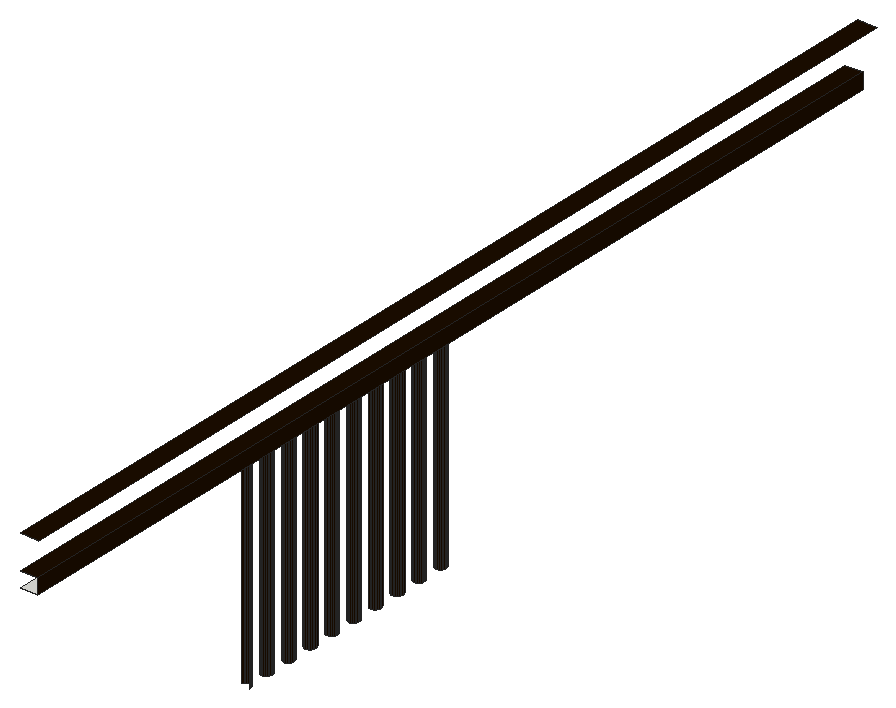
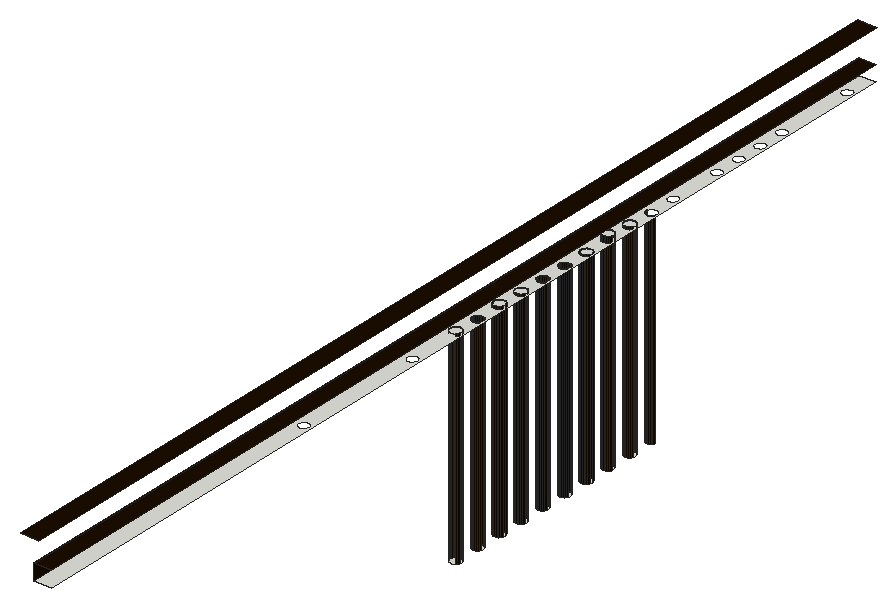
# SketchUp Ruby script. Lengths in inches.
U = 1.inch
M = Sketchup.active_model
def pt(a) = Geom::Point3d.new(a.map { |v| v * U })
def face(e, loops, mat)
  f = e.add_face(loops[0].map { |a| pt(a) })
  loops[1..].each { |l| e.add_face(l.map { |a| pt(a) }).erase! }
  f.material = f.back_material = mat if mat
  f
end
# faces: each face lists its corners as indices into pts; further lists are holes
def faces(e, pts, list, mat = nil) = list.each { |f| face(e, (f[0].is_a?(Array) ? f : [f]).map { |l| l.map { |i| pts[i] } }, mat) }
# xy, xz, yz: faces in a plane at the given z, y or x. An outline is a flat list of corners, or four numbers for a rectangle; further outlines are holes
def ring(l) = l.size == 4 ? [[l[0], l[1]], [l[2], l[1]], [l[2], l[3]], [l[0], l[3]]] : l.each_slice(2).to_a
def flat(e, list, mat, &to3) = list.each { |f| face(e, (f[0].is_a?(Array) ? f : [f]).map { |l| ring(l).map { |u, v| to3.(u, v) } }, mat) }
def xy(e, z, list, mat = nil) = flat(e, list, mat) { |x, y| [x, y, z] }
def xz(e, y, list, mat = nil) = flat(e, list, mat) { |x, z| [x, y, z] }
def yz(e, x, list, mat = nil) = flat(e, list, mat) { |y, z| [x, y, z] }
def lines(e, pts, list) = list.each { |a, b| e.add_line(pt(pts[a]), pt(pts[b])) }
# prism: a flat outline (further loops are holes) pulled along v
def prism(e, loops, v, mat = nil)
  f = face(e, loops, mat); d = Geom::Vector3d.new(v.map { |x| x * U })
  f.pushpull(f.normal.samedirection?(d) ? d.length : -d.length)
end
def box(e, o, s, mat = nil) = prism(e, [[o, [o[0] + s[0], o[1], o[2]], [o[0] + s[0], o[1] + s[1], o[2]], [o[0], o[1] + s[1], o[2]]]], [0, 0, s[2]], mat)
def at(x, y, z, deg = 0) = Geom::Transformation.translation(pt([x, y, z])) * Geom::Transformation.rotation(ORIGIN, Z_AXIS, deg.degrees)
def axes(o, x, y, z) = Geom::Transformation.new([*x, 0, *y, 0, *z, 0, *pt(o).to_a, 1])
def part(name) = M.definitions.add(name)
# library, detail: a bought-in or finely detailed component or shape, given as its bounding box
def library(name, o, s) = part(name).tap { |d| box(d.entities, o, s) }
def detail(e, o, s) = box(e.add_group.entities, o, s)
def put(e, d, t, mat = nil) = e.add_instance(d, t).tap { |i| i.material = mat if mat }
def group(e, t, mat = nil) = e.add_group.tap { |g| g.transformation = t; g.material = mat if mat }.entities
root = M.entities
M.materials.add("[Metal Seamed]1").color = [28, 14, 0]
xy(root,618.25,[[363.55,142.79,363.21,142.87,362.92,143.04,362.67,143.28,362.5,143.58,362.41,143.91,362.41,144.25,362.5,144.58,362.67,144.88,362.91,145.125,363.2,145.3,363.54,145.39,363.88,145.39,364.21,145.3,364.51,145.13,364.75,144.89,364.92,144.59,365.01,144.26,365.01,143.92,364.93,143.59,364.76,143.29,364.51,143.05,364.22,142.875,363.89,142.79],[363.55,149.22,363.21,149.31,362.92,149.48,362.67,149.72,362.5,150.02,362.41,150.35,362.41,150.69,362.5,151.02,362.67,151.32,362.91,151.5625,363.2,151.74,363.54,151.83,363.88,151.83,364.21,151.74,364.51,151.57,364.75,151.33,364.92,151.03,365.01,150.7,365.01,150.36,364.93,150.03,364.76,149.73,364.51,149.49,364.22,149.3125,363.89,149.22],[363.55,155.66,363.21,155.75,362.92,155.92,362.67,156.16,362.5,156.46,362.41,156.79,362.41,157.13,362.5,157.46,362.67,157.76,362.91,158,363.2,158.17,363.54,158.26,363.88,158.26,364.21,158.18,364.51,158.01,364.75,157.76,364.92,157.47,365.01,157.14,365.01,156.8,364.93,156.46,364.76,156.17,364.51,155.92,364.22,155.75,363.89,155.66],[363.55,162.1,363.21,162.19,362.92,162.36,362.67,162.6,362.5,162.89,362.41,163.22,362.41,163.57,362.5,163.9,362.67,164.19,362.91,164.4375,363.2,164.61,363.54,164.7,363.88,164.7,364.21,164.61,364.51,164.44,364.75,164.2,364.92,163.91,365.01,163.58,365.01,163.23,364.93,162.9,364.76,162.6,364.51,162.36,364.22,162.1875,363.89,162.1],[363.55,168.54,363.21,168.62,362.92,168.79,362.67,169.03,362.5,169.33,362.41,169.66,362.41,170,362.5,170.33,362.67,170.63,362.91,170.875,363.2,171.05,363.54,171.14,363.88,171.14,364.21,171.05,364.51,170.88,364.75,170.64,364.92,170.34,365.01,170.01,365.01,169.67,364.93,169.34,364.76,169.04,364.51,168.8,364.22,168.625,363.89,168.54],
  [363.55,174.97,363.21,175.06,362.92,175.23,362.67,175.47,362.5,175.77,362.41,176.1,362.41,176.44,362.5,176.77,362.67,177.07,362.91,177.3125,363.2,177.49,363.54,177.58,363.88,177.58,364.21,177.49,364.51,177.32,364.75,177.08,364.92,176.78,365.01,176.45,365.01,176.11,364.93,175.78,364.76,175.48,364.51,175.24,364.22,175.0625,363.89,174.97],[363.55,181.41,363.21,181.5,362.92,181.67,362.67,181.91,362.5,182.21,362.41,182.54,362.41,182.88,362.5,183.21,362.67,183.51,362.91,183.75,363.2,183.92,363.54,184.01,363.88,184.01,364.21,183.93,364.51,183.76,364.75,183.51,364.92,183.22,365.01,182.89,365.01,182.55,364.93,182.21,364.76,181.92,364.51,181.67,364.22,181.5,363.89,181.41],[363.55,187.85,363.21,187.94,362.92,188.11,362.67,188.35,362.5,188.64,362.41,188.97,362.41,189.32,362.5,189.65,362.67,189.94,362.91,190.1875,363.2,190.36,363.54,190.45,363.88,190.45,364.21,190.36,364.51,190.19,364.75,189.95,364.92,189.66,365.01,189.33,365.01,188.98,364.93,188.65,364.76,188.35,364.51,188.11,364.22,187.9375,363.89,187.85],[363.55,194.29,363.21,194.37,362.92,194.54,362.67,194.78,362.5,195.08,362.41,195.41,362.41,195.75,362.5,196.08,362.67,196.38,362.91,196.625,363.2,196.8,363.54,196.89,363.88,196.89,364.21,196.8,364.51,196.63,364.75,196.39,364.92,196.09,365.01,195.76,365.01,195.42,364.93,195.09,364.76,194.79,364.51,194.55,364.22,194.375,363.89,194.29]])
xy(root,666.66,[[[361.98,73.28,366.15,317.52],[363.55,78.41,363.89,78.41,364.22,78.5,364.51,78.67,364.76,78.92,364.93,79.21,365.01,79.55,365.01,79.89,364.92,80.22,364.75,80.51,364.51,80.76,364.21,80.93,363.88,81.01,363.54,81.01,363.2,80.92,362.91,80.75,362.67,80.51,362.5,80.21,362.41,79.88,362.41,79.54,362.5,79.21,362.67,78.91,362.92,78.67,363.21,78.5],[363.55,97.72,363.89,97.72,364.22,97.8125,364.51,97.99,364.76,98.23,364.93,98.53,365.01,98.86,365.01,99.2,364.92,99.53,364.75,99.83,364.51,100.07,364.21,100.24,363.88,100.33,363.54,100.33,363.2,100.24,362.91,100.0625,362.67,99.82,362.5,99.52,362.41,99.19,362.41,98.85,362.5,98.52,362.67,98.22,362.92,97.98,363.21,97.81],[363.55,104.16,363.89,104.16,364.22,104.25,364.51,104.42,364.76,104.67,364.93,104.96,365.01,105.3,365.01,105.64,364.92,105.97,364.75,106.26,364.51,106.51,364.21,106.68,363.88,106.76,363.54,106.76,363.2,106.67,362.91,106.5,362.67,106.26,362.5,105.96,362.41,105.63,362.41,105.29,362.5,104.96,362.67,104.66,362.92,104.42,363.21,104.25],[363.55,110.6,363.89,110.6,364.22,110.6875,364.51,110.86,364.76,111.1,364.93,111.4,365.01,111.73,365.01,112.08,364.92,112.41,364.75,112.7,364.51,112.94,364.21,113.11,363.88,113.2,363.54,113.2,363.2,113.11,362.91,112.9375,362.67,112.69,362.5,112.4,362.41,112.07,362.41,111.72,362.5,111.39,362.67,111.1,362.92,110.86,363.21,110.69],[363.55,117.04,363.89,117.04,364.22,117.125,364.51,117.3,364.76,117.54,364.93,117.84,365.01,118.17,365.01,118.51,364.92,118.84,364.75,119.14,364.51,119.38,364.21,119.55,363.88,119.64,363.54,119.64,363.2,119.55,362.91,119.375,362.67,119.13,362.5,118.83,362.41,118.5,362.41,118.16,362.5,117.83,362.67,117.53,362.92,117.29,363.21,117.12],[363.55,129.91,363.89,129.91,364.22,130,364.51,130.17,364.76,130.42,364.93,130.71,365.01,131.05,365.01,131.39,364.92,131.72,364.75,132.01,364.51,132.26,364.21,132.43,363.88,132.51,363.54,132.51,363.2,132.42,362.91,132.25,362.67,132.01,362.5,131.71,362.41,131.38,362.41,131.04,362.5,130.71,362.67,130.41,362.92,130.17,363.21,130],[363.55,136.35,363.89,136.35,364.22,136.4375,364.51,136.61,364.76,136.85,364.93,137.15,365.01,137.48,365.01,137.83,364.92,138.16,364.75,138.45,364.51,138.69,364.21,138.86,363.88,138.95,363.54,138.95,363.2,138.86,362.91,138.6875,362.67,138.44,362.5,138.15,362.41,137.82,362.41,137.47,362.5,137.14,362.67,136.85,362.92,136.61,363.21,136.44],[363.55,162.1,363.89,162.1,364.22,162.1875,364.51,162.36,364.76,162.6,364.93,162.9,365.01,163.23,365.01,163.58,364.92,163.91,364.75,164.2,364.51,164.44,364.21,164.61,363.88,164.7,363.54,164.7,363.2,164.61,362.91,164.4375,362.67,164.19,362.5,163.9,362.41,163.57,362.41,163.22,362.5,162.89,362.67,162.6,362.92,162.36,363.21,162.19],[363.55,168.54,363.89,168.54,364.22,168.625,364.51,168.8,364.76,169.04,364.93,169.34,365.01,169.67,365.01,170.01,364.92,170.34,364.75,170.64,364.51,170.88,364.21,171.05,363.88,171.14,363.54,171.14,363.2,171.05,362.91,170.875,362.67,170.63,362.5,170.33,362.41,170,362.41,169.66,362.5,169.33,362.67,169.03,362.92,168.79,363.21,168.62],[363.55,187.85,363.89,187.85,364.22,187.9375,364.51,188.11,364.76,188.35,364.93,188.65,365.01,188.98,365.01,189.33,364.92,189.66,364.75,189.95,364.51,190.19,364.21,190.36,363.88,190.45,363.54,190.45,363.2,190.36,362.91,190.1875,362.67,189.94,362.5,189.65,362.41,189.32,362.41,188.97,362.5,188.64,362.67,188.35,362.92,188.11,363.21,187.94],[363.55,207.16,363.89,207.16,364.22,207.25,364.51,207.42,364.76,207.67,364.93,207.96,365.01,208.3,365.01,208.64,364.92,208.97,364.75,209.26,364.51,209.51,364.21,209.68,363.88,209.76,363.54,209.76,363.2,209.67,362.91,209.5,362.67,209.26,362.5,208.96,362.41,208.63,362.41,208.29,362.5,207.96,362.67,207.66,362.92,207.42,363.21,207.25],[363.55,239.35,363.89,239.35,364.22,239.4375,364.51,239.61,364.76,239.85,364.93,240.15,365.01,240.48,365.01,240.83,364.92,241.16,364.75,241.45,364.51,241.69,364.21,241.86,363.88,241.95,363.54,241.95,363.2,241.86,362.91,241.6875,362.67,241.44,362.5,241.15,362.41,240.82,362.41,240.47,362.5,240.14,362.67,239.85,362.92,239.61,363.21,239.44]]])
xy(root,666.8125,[[363.55,155.66,363.89,155.66,364.22,155.75,364.51,155.92,364.76,156.17,364.93,156.46,365.01,156.8,365.01,157.14,364.92,157.47,364.75,157.76,364.51,158.01,364.21,158.18,363.88,158.26,363.54,158.26,363.2,158.17,362.91,158,362.67,157.76,362.5,157.46,362.41,157.13,362.41,156.79,362.5,156.46,362.67,156.16,362.92,155.92,363.21,155.75]])
xy(root,667,[[363.55,174.97,363.89,174.97,364.22,175.0625,364.51,175.24,364.76,175.48,364.93,175.78,365.01,176.11,365.01,176.45,364.92,176.78,364.75,177.08,364.51,177.32,364.21,177.49,363.88,177.58,363.54,177.58,363.2,177.49,362.91,177.3125,362.67,177.07,362.5,176.77,362.41,176.44,362.41,176.1,362.5,175.77,362.67,175.47,362.92,175.23,363.21,175.06]])
xy(root,667.125,[[363.55,142.79,363.89,142.79,364.22,142.875,364.51,143.05,364.76,143.29,364.93,143.59,365.01,143.92,365.01,144.26,364.92,144.59,364.75,144.89,364.51,145.13,364.21,145.3,363.88,145.39,363.54,145.39,363.2,145.3,362.91,145.125,362.67,144.88,362.5,144.58,362.41,144.25,362.41,143.91,362.5,143.58,362.67,143.28,362.92,143.04,363.21,142.87],[363.55,194.29,363.89,194.29,364.22,194.375,364.51,194.55,364.76,194.79,364.93,195.09,365.01,195.42,365.01,195.76,364.92,196.09,364.75,196.39,364.51,196.63,364.21,196.8,363.88,196.89,363.54,196.89,363.2,196.8,362.91,196.625,362.67,196.38,362.5,196.08,362.41,195.75,362.41,195.41,362.5,195.08,362.67,194.78,362.92,194.54,363.21,194.37]])
xy(root,667.25,[[363.55,181.41,363.89,181.41,364.22,181.5,364.51,181.67,364.76,181.92,364.93,182.21,365.01,182.55,365.01,182.89,364.92,183.22,364.75,183.51,364.51,183.76,364.21,183.93,363.88,184.01,363.54,184.01,363.2,183.92,362.91,183.75,362.67,183.51,362.5,183.21,362.41,182.88,362.41,182.54,362.5,182.21,362.67,181.91,362.92,181.67,363.21,181.5]])
xy(root,667.9375,[[363.55,149.22,363.89,149.22,364.22,149.3125,364.51,149.49,364.76,149.73,364.93,150.03,365.01,150.36,365.01,150.7,364.92,151.03,364.75,151.33,364.51,151.57,364.21,151.74,363.88,151.83,363.54,151.83,363.2,151.74,362.91,151.5625,362.67,151.32,362.5,151.02,362.41,150.69,362.41,150.35,362.5,150.02,362.67,149.72,362.92,149.48,363.21,149.31]])
xy(root,670.37,[[361.98,73.28,366.15,317.52]],"[Metal Seamed]1")
xy(root,678.3125,[[361.97,73.28,366.34,321.28]],"[Metal Seamed]1")
xz(root,138.95,[[363.54,618.25,363.88,666.66]],"[Metal Seamed]1")
xz(root,142.79,[[363.55,618.25,363.89,667.125]],"[Metal Seamed]1")
xz(root,145.39,[[363.54,618.25,363.88,667.125]],"[Metal Seamed]1")
xz(root,149.22,[[363.55,618.25,363.89,667.9375]],"[Metal Seamed]1")
xz(root,151.83,[[363.54,618.25,363.88,667.9375]],"[Metal Seamed]1")
xz(root,155.66,[[363.55,618.25,363.89,666.8125]],"[Metal Seamed]1")
xz(root,158.26,[[363.54,618.25,363.88,666.8125]],"[Metal Seamed]1")
xz(root,162.1,[[363.55,618.25,363.89,666.66]],"[Metal Seamed]1")
xz(root,164.7,[[363.54,618.25,363.88,666.66]],"[Metal Seamed]1")
xz(root,168.54,[[363.55,618.25,363.89,666.66]],"[Metal Seamed]1")
xz(root,171.14,[[363.54,618.25,363.88,666.66]],"[Metal Seamed]1")
xz(root,174.97,[[363.55,618.25,363.89,667]],"[Metal Seamed]1")
xz(root,177.58,[[363.54,618.25,363.88,667]],"[Metal Seamed]1")
xz(root,181.41,[[363.55,618.25,363.89,667.25]],"[Metal Seamed]1")
xz(root,184.01,[[363.54,618.25,363.88,667.25]],"[Metal Seamed]1")
xz(root,187.85,[[363.55,618.25,363.89,666.66]],"[Metal Seamed]1")
xz(root,190.45,[[363.54,618.25,363.88,666.66]],"[Metal Seamed]1")
xz(root,194.29,[[363.55,618.25,363.89,667.125]],"[Metal Seamed]1")
yz(root,365.01,[[137.48,618.25,137.83,666.66],[143.92,618.25,144.26,667.125],[150.36,618.25,150.7,667.9375],[156.8,618.25,157.14,666.8125],[163.23,618.25,163.58,666.66],
  [169.67,618.25,170.01,666.66],[176.11,618.25,176.45,667],[182.55,618.25,182.89,667.25],[188.98,618.25,189.33,666.66],[195.42,618.25,195.76,667.125]],"[Metal Seamed]1")
yz(root,366.15,[[73.28,666.66,317.52,670.37]],"[Metal Seamed]1")
p = [[365.01,137.83,618.25],[364.92,138.16,618.25],[364.92,138.16,666.66],[365.01,137.83,666.66],[362.67,138.44,618.25],[362.5,138.15,618.25],
  [362.5,138.15,666.66],[362.67,138.44,666.66],[364.75,138.45,618.25],[364.75,138.45,666.66],[362.91,138.6875,618.25],[362.91,138.6875,666.66],
  [364.51,138.69,618.25],[364.51,138.69,666.66],[363.2,138.86,618.25],[363.2,138.86,666.66],[364.21,138.86,618.25],[364.21,138.86,666.66],
  [363.54,138.95,618.25],[363.54,138.95,666.66],[363.88,138.95,618.25],[363.88,138.95,666.66],[363.21,142.87,618.25],[363.55,142.79,618.25],
  [363.55,142.79,667.125],[363.21,142.87,667.125],[363.89,142.79,618.25],[364.22,142.875,618.25],[364.22,142.875,667.125],[363.89,142.79,667.125],
  [362.92,143.04,618.25],[362.92,143.04,667.125],[364.51,143.05,618.25],[364.51,143.05,667.125],[362.67,143.28,618.25],[362.67,143.28,667.125],
  [364.76,143.29,618.25],[364.76,143.29,667.125],[362.5,143.58,618.25],[362.5,143.58,667.125],[364.93,143.59,618.25],[364.93,143.59,667.125],
  [365.01,143.92,618.25],[365.01,143.92,667.125],[365.01,144.26,618.25],[364.92,144.59,618.25],[364.92,144.59,667.125],[365.01,144.26,667.125],
  [362.67,144.88,618.25],[362.5,144.58,618.25],[362.5,144.58,667.125],[362.67,144.88,667.125],[364.75,144.89,618.25],[364.75,144.89,667.125],
  [362.91,145.125,618.25],[362.91,145.125,667.125],[364.51,145.13,618.25],[364.51,145.13,667.125],[363.2,145.3,618.25],[363.2,145.3,667.125],
  [364.21,145.3,618.25],[364.21,145.3,667.125],[363.54,145.39,618.25],[363.54,145.39,667.125],[363.88,145.39,618.25],[363.88,145.39,667.125],
  [363.21,149.31,618.25],[363.55,149.22,618.25],[363.55,149.22,667.9375],[363.21,149.31,667.9375],[363.89,149.22,618.25],[364.22,149.3125,618.25],
  [364.22,149.3125,667.9375],[363.89,149.22,667.9375],[362.92,149.48,618.25],[362.92,149.48,667.9375],[364.51,149.49,618.25],[364.51,149.49,667.9375],
  [362.67,149.72,618.25],[362.67,149.72,667.9375],[364.76,149.73,618.25],[364.76,149.73,667.9375],[362.5,150.02,618.25],[362.5,150.02,667.9375],
  [364.93,150.03,618.25],[364.93,150.03,667.9375],[365.01,150.36,618.25],[365.01,150.36,667.9375],[365.01,150.7,618.25],[364.92,151.03,618.25],
  [364.92,151.03,667.9375],[365.01,150.7,667.9375],[362.67,151.32,618.25],[362.5,151.02,618.25],[362.5,151.02,667.9375],[362.67,151.32,667.9375],
  [364.75,151.33,618.25],[364.75,151.33,667.9375],[362.91,151.5625,618.25],[362.91,151.5625,667.9375],[364.51,151.57,618.25],[364.51,151.57,667.9375],
  [363.2,151.74,618.25],[363.2,151.74,667.9375],[364.21,151.74,618.25],[364.21,151.74,667.9375],[363.54,151.83,618.25],[363.54,151.83,667.9375],
  [363.88,151.83,618.25],[363.88,151.83,667.9375],[362.92,155.92,618.25],[363.21,155.75,618.25],[363.21,155.75,666.8125],[362.92,155.92,666.8125],
  [363.55,155.66,618.25],[363.55,155.66,666.8125],[363.89,155.66,618.25],[364.22,155.75,618.25],[364.22,155.75,666.8125],[363.89,155.66,666.8125],
  [364.51,155.92,618.25],[364.51,155.92,666.8125],[362.67,156.16,618.25],[362.67,156.16,666.8125],[364.76,156.17,618.25],[364.76,156.17,666.8125],
  [362.5,156.46,618.25],[362.5,156.46,666.8125],[364.93,156.46,618.25],[364.93,156.46,666.8125],[365.01,156.8,618.25],[365.01,156.8,666.8125],
  [365.01,157.14,618.25],[364.92,157.47,618.25],[364.92,157.47,666.8125],[365.01,157.14,666.8125],[362.67,157.76,618.25],[362.5,157.46,618.25],
  [362.5,157.46,666.8125],[362.67,157.76,666.8125],[364.75,157.76,618.25],[364.75,157.76,666.8125],[362.91,158,618.25],[362.91,158,666.8125],
  [364.51,158.01,618.25],[364.51,158.01,666.8125],[363.2,158.17,618.25],[363.2,158.17,666.8125],[364.21,158.18,618.25],[364.21,158.18,666.8125],
  [363.54,158.26,618.25],[363.54,158.26,666.8125],[363.88,158.26,618.25],[363.88,158.26,666.8125],[363.21,162.19,618.25],[363.55,162.1,618.25],
  [363.55,162.1,666.66],[363.21,162.19,666.66],[363.89,162.1,618.25],[364.22,162.1875,618.25],[364.22,162.1875,666.66],[363.89,162.1,666.66],
  [362.92,162.36,618.25],[362.92,162.36,666.66],[364.51,162.36,618.25],[364.51,162.36,666.66],[362.67,162.6,618.25],[362.67,162.6,666.66],
  [364.76,162.6,618.25],[364.76,162.6,666.66],[362.5,162.89,618.25],[362.5,162.89,666.66],[364.93,162.9,618.25],[364.93,162.9,666.66],
  [365.01,163.23,618.25],[365.01,163.23,666.66],[365.01,163.58,618.25],[364.92,163.91,618.25],[364.92,163.91,666.66],[365.01,163.58,666.66],
  [362.67,164.19,618.25],[362.5,163.9,618.25],[362.5,163.9,666.66],[362.67,164.19,666.66],[364.75,164.2,618.25],[364.75,164.2,666.66],
  [362.91,164.4375,618.25],[362.91,164.4375,666.66],[364.51,164.44,618.25],[364.51,164.44,666.66],[363.2,164.61,618.25],[363.2,164.61,666.66],
  [364.21,164.61,618.25],[364.21,164.61,666.66],[363.54,164.7,618.25],[363.54,164.7,666.66],[363.88,164.7,618.25],[363.88,164.7,666.66],
  [363.21,168.62,618.25],[363.55,168.54,618.25],[363.55,168.54,666.66],[363.21,168.62,666.66],[363.89,168.54,618.25],[364.22,168.625,618.25],
  [364.22,168.625,666.66],[363.89,168.54,666.66],[362.92,168.79,618.25],[362.92,168.79,666.66],[364.51,168.8,618.25],[364.51,168.8,666.66],
  [362.67,169.03,618.25],[362.67,169.03,666.66],[364.76,169.04,618.25],[364.76,169.04,666.66],[362.5,169.33,618.25],[362.5,169.33,666.66],
  [364.93,169.34,618.25],[364.93,169.34,666.66],[365.01,169.67,618.25],[365.01,169.67,666.66],[365.01,170.01,618.25],[364.92,170.34,618.25],
  [364.92,170.34,666.66],[365.01,170.01,666.66],[362.67,170.63,618.25],[362.5,170.33,618.25],[362.5,170.33,666.66],[362.67,170.63,666.66],
  [364.75,170.64,618.25],[364.75,170.64,666.66],[362.91,170.875,618.25],[362.91,170.875,666.66],[364.51,170.88,618.25],[364.51,170.88,666.66],
  [363.2,171.05,618.25],[363.2,171.05,666.66],[364.21,171.05,618.25],[364.21,171.05,666.66],[363.54,171.14,618.25],[363.54,171.14,666.66],
  [363.88,171.14,618.25],[363.88,171.14,666.66],[363.21,175.06,618.25],[363.55,174.97,618.25],[363.55,174.97,667],[363.21,175.06,667],
  [363.89,174.97,618.25],[364.22,175.0625,618.25],[364.22,175.0625,667],[363.89,174.97,667],[362.92,175.23,618.25],[362.92,175.23,667],
  [364.51,175.24,618.25],[364.51,175.24,667],[362.67,175.47,618.25],[362.67,175.47,667],[364.76,175.48,618.25],[364.76,175.48,667],
  [362.5,175.77,618.25],[362.5,175.77,667],[364.93,175.78,618.25],[364.93,175.78,667],[365.01,176.11,618.25],[365.01,176.11,667],
  [365.01,176.45,618.25],[364.92,176.78,618.25],[364.92,176.78,667],[365.01,176.45,667],[362.67,177.07,618.25],[362.5,176.77,618.25],
  [362.5,176.77,667],[362.67,177.07,667],[364.75,177.08,618.25],[364.75,177.08,667],[362.91,177.3125,618.25],[362.91,177.3125,667],
  [364.51,177.32,618.25],[364.51,177.32,667],[363.2,177.49,618.25],[363.2,177.49,667],[364.21,177.49,618.25],[364.21,177.49,667],
  [363.54,177.58,618.25],[363.54,177.58,667],[363.88,177.58,618.25],[363.88,177.58,667],[363.21,181.5,618.25],[363.55,181.41,618.25],
  [363.55,181.41,667.25],[363.21,181.5,667.25],[363.89,181.41,618.25],[364.22,181.5,618.25],[364.22,181.5,667.25],[363.89,181.41,667.25],
  [362.92,181.67,618.25],[362.92,181.67,667.25],[364.51,181.67,618.25],[364.51,181.67,667.25],[362.67,181.91,618.25],[362.67,181.91,667.25],
  [364.76,181.92,618.25],[364.76,181.92,667.25],[362.5,182.21,618.25],[362.5,182.21,667.25],[364.93,182.21,618.25],[364.93,182.21,667.25],
  [365.01,182.55,618.25],[365.01,182.55,667.25],[365.01,182.89,618.25],[364.92,183.22,618.25],[364.92,183.22,667.25],[365.01,182.89,667.25],
  [362.67,183.51,618.25],[362.5,183.21,618.25],[362.5,183.21,667.25],[362.67,183.51,667.25],[364.75,183.51,618.25],[364.75,183.51,667.25],
  [362.91,183.75,618.25],[362.91,183.75,667.25],[364.51,183.76,618.25],[364.51,183.76,667.25],[363.2,183.92,618.25],[363.2,183.92,667.25],
  [364.21,183.93,618.25],[364.21,183.93,667.25],[363.54,184.01,618.25],[363.54,184.01,667.25],[363.88,184.01,618.25],[363.88,184.01,667.25],
  [363.21,187.94,618.25],[363.55,187.85,618.25],[363.55,187.85,666.66],[363.21,187.94,666.66],[363.89,187.85,618.25],[364.22,187.9375,618.25],
  [364.22,187.9375,666.66],[363.89,187.85,666.66],[362.92,188.11,618.25],[362.92,188.11,666.66],[364.51,188.11,618.25],[364.51,188.11,666.66],
  [362.67,188.35,618.25],[362.67,188.35,666.66],[364.76,188.35,618.25],[364.76,188.35,666.66],[362.5,188.64,618.25],[362.5,188.64,666.66],
  [364.93,188.65,618.25],[364.93,188.65,666.66],[365.01,188.98,618.25],[365.01,188.98,666.66],[365.01,189.33,618.25],[364.92,189.66,618.25],
  [364.92,189.66,666.66],[365.01,189.33,666.66],[362.67,189.94,618.25],[362.5,189.65,618.25],[362.5,189.65,666.66],[362.67,189.94,666.66],
  [364.75,189.95,618.25],[364.75,189.95,666.66],[362.91,190.1875,618.25],[362.91,190.1875,666.66],[364.51,190.19,618.25],[364.51,190.19,666.66],
  [363.2,190.36,618.25],[363.2,190.36,666.66],[364.21,190.36,618.25],[364.21,190.36,666.66],[363.54,190.45,618.25],[363.54,190.45,666.66],
  [363.88,190.45,618.25],[363.88,190.45,666.66],[363.21,194.37,618.25],[363.55,194.29,618.25],[363.55,194.29,667.125],[363.21,194.37,667.125],
  [363.89,194.29,618.25],[364.22,194.375,618.25],[364.22,194.375,667.125],[363.89,194.29,667.125],[362.92,194.54,618.25],[362.92,194.54,667.125],
  [364.51,194.55,618.25],[364.51,194.55,667.125],[362.67,194.78,618.25],[362.67,194.78,667.125],[364.76,194.79,618.25],[364.76,194.79,667.125],
  [362.5,195.08,618.25],[362.5,195.08,667.125],[364.93,195.09,618.25],[364.93,195.09,667.125],[365.01,195.42,618.25],[365.01,195.42,667.125],
  [365.01,195.76,618.25],[364.92,196.09,618.25],[364.92,196.09,667.125],[365.01,195.76,667.125],[362.67,196.38,618.25],[362.5,196.08,618.25],
  [362.5,196.08,667.125],[362.67,196.38,667.125],[364.75,196.39,618.25],[364.75,196.39,667.125],[362.91,196.625,618.25],[362.91,196.625,667.125],
  [364.51,196.63,618.25],[364.51,196.63,667.125]]
faces(root,p,[[0,1,2,3],[4,5,6,7],[1,8,9,2],[10,4,7,11],[8,12,13,9],[14,10,11,15],[12,16,17,13],[18,14,15,19],
  [16,20,21,17],[22,23,24,25],[26,27,28,29],[30,22,25,31],[27,32,33,28],[34,30,31,35],[32,36,37,33],[38,34,35,39],
  [36,40,41,37],[40,42,43,41],[44,45,46,47],[48,49,50,51],[45,52,53,46],[54,48,51,55],[52,56,57,53],[58,54,55,59],
  [56,60,61,57],[62,58,59,63],[60,64,65,61],[66,67,68,69],[70,71,72,73],[74,66,69,75],[71,76,77,72],[78,74,75,79],
  [76,80,81,77],[82,78,79,83],[80,84,85,81],[84,86,87,85],[88,89,90,91],[92,93,94,95],[89,96,97,90],[98,92,95,99],
  [96,100,101,97],[102,98,99,103],[100,104,105,101],[106,102,103,107],[104,108,109,105],[110,111,112,113],[111,114,115,112],[116,117,118,119],
  [117,120,121,118],[122,110,113,123],[120,124,125,121],[126,122,123,127],[124,128,129,125],[128,130,131,129],[132,133,134,135],[136,137,138,139],
  [133,140,141,134],[142,136,139,143],[140,144,145,141],[146,142,143,147],[144,148,149,145],[150,146,147,151],[148,152,153,149],[154,155,156,157],
  [158,159,160,161],[162,154,157,163],[159,164,165,160],[166,162,163,167],[164,168,169,165],[170,166,167,171],[168,172,173,169],[172,174,175,173],
  [176,177,178,179],[180,181,182,183],[177,184,185,178],[186,180,183,187],[184,188,189,185],[190,186,187,191],[188,192,193,189],[194,190,191,195],
  [192,196,197,193],[198,199,200,201],[202,203,204,205],[206,198,201,207],[203,208,209,204],[210,206,207,211],[208,212,213,209],[214,210,211,215],
  [212,216,217,213],[216,218,219,217],[220,221,222,223],[224,225,226,227],[221,228,229,222],[230,224,227,231],[228,232,233,229],[234,230,231,235],
  [232,236,237,233],[238,234,235,239],[236,240,241,237],[242,243,244,245],[246,247,248,249],[250,242,245,251],[247,252,253,248],[254,250,251,255],
  [252,256,257,253],[258,254,255,259],[256,260,261,257],[260,262,263,261],[264,265,266,267],[268,269,270,271],[265,272,273,266],[274,268,271,275],
  [272,276,277,273],[278,274,275,279],[276,280,281,277],[282,278,279,283],[280,284,285,281],[286,287,288,289],[290,291,292,293],[294,286,289,295],
  [291,296,297,292],[298,294,295,299],[296,300,301,297],[302,298,299,303],[300,304,305,301],[304,306,307,305],[308,309,310,311],[312,313,314,315],
  [309,316,317,310],[318,312,315,319],[316,320,321,317],[322,318,319,323],[320,324,325,321],[326,322,323,327],[324,328,329,325],[330,331,332,333],
  [334,335,336,337],[338,330,333,339],[335,340,341,336],[342,338,339,343],[340,344,345,341],[346,342,343,347],[344,348,349,345],[348,350,351,349],
  [352,353,354,355],[356,357,358,359],[353,360,361,354],[362,356,359,363],[360,364,365,361],[366,362,363,367],[364,368,369,365],[370,366,367,371],
  [368,372,373,369],[374,375,376,377],[378,379,380,381],[382,374,377,383],[379,384,385,380],[386,382,383,387],[384,388,389,385],[390,386,387,391],
  [388,392,393,389],[392,394,395,393],[396,397,398,399],[400,401,402,403],[397,404,405,398],[406,400,403,407],[404,408,409,405]],"[Metal Seamed]1")
